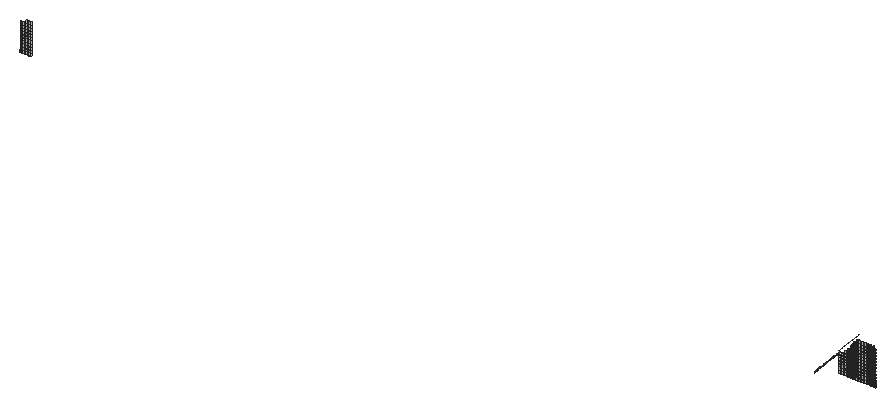
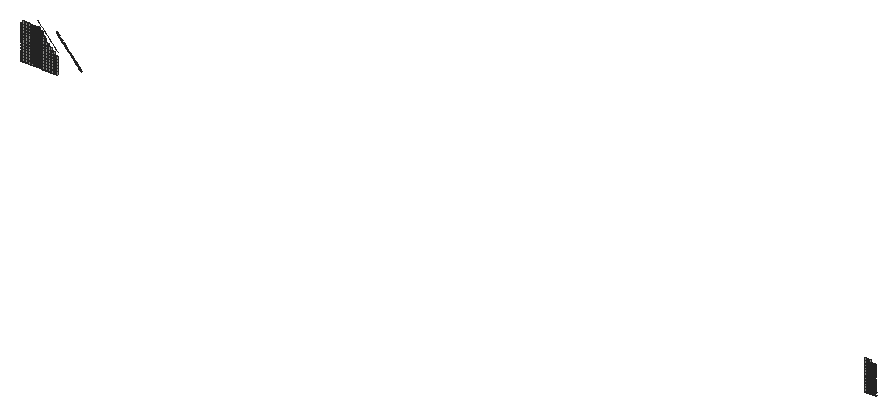
# SketchUp Ruby script. Lengths in inches.
U = 1.inch
M = Sketchup.active_model
def pt(a) = Geom::Point3d.new(a.map { |v| v * U })
def face(e, loops, mat)
  f = e.add_face(loops[0].map { |a| pt(a) })
  loops[1..].each { |l| e.add_face(l.map { |a| pt(a) }).erase! }
  f.material = f.back_material = mat if mat
  f
end
# faces: each face lists its corners as indices into pts; further lists are holes
def faces(e, pts, list, mat = nil) = list.each { |f| face(e, (f[0].is_a?(Array) ? f : [f]).map { |l| l.map { |i| pts[i] } }, mat) }
# xy, xz, yz: faces in a plane at the given z, y or x. An outline is a flat list of corners, or four numbers for a rectangle; further outlines are holes
def ring(l) = l.size == 4 ? [[l[0], l[1]], [l[2], l[1]], [l[2], l[3]], [l[0], l[3]]] : l.each_slice(2).to_a
def flat(e, list, mat, &to3) = list.each { |f| face(e, (f[0].is_a?(Array) ? f : [f]).map { |l| ring(l).map { |u, v| to3.(u, v) } }, mat) }
def xy(e, z, list, mat = nil) = flat(e, list, mat) { |x, y| [x, y, z] }
def xz(e, y, list, mat = nil) = flat(e, list, mat) { |x, z| [x, y, z] }
def yz(e, x, list, mat = nil) = flat(e, list, mat) { |y, z| [x, y, z] }
def lines(e, pts, list) = list.each { |a, b| e.add_line(pt(pts[a]), pt(pts[b])) }
# prism: a flat outline (further loops are holes) pulled along v
def prism(e, loops, v, mat = nil)
  f = face(e, loops, mat); d = Geom::Vector3d.new(v.map { |x| x * U })
  f.pushpull(f.normal.samedirection?(d) ? d.length : -d.length)
end
def box(e, o, s, mat = nil) = prism(e, [[o, [o[0] + s[0], o[1], o[2]], [o[0] + s[0], o[1] + s[1], o[2]], [o[0], o[1] + s[1], o[2]]]], [0, 0, s[2]], mat)
def at(x, y, z, deg = 0) = Geom::Transformation.translation(pt([x, y, z])) * Geom::Transformation.rotation(ORIGIN, Z_AXIS, deg.degrees)
def axes(o, x, y, z) = Geom::Transformation.new([*x, 0, *y, 0, *z, 0, *pt(o).to_a, 1])
def part(name) = M.definitions.add(name)
# library, detail: a bought-in or finely detailed component or shape, given as its bounding box
def library(name, o, s) = part(name).tap { |d| box(d.entities, o, s) }
def detail(e, o, s) = box(e.add_group.entities, o, s)
def put(e, d, t, mat = nil) = e.add_instance(d, t).tap { |i| i.material = mat if mat }
def group(e, t, mat = nil) = e.add_group.tap { |g| g.transformation = t; g.material = mat if mat }.entities
root = M.entities
M.materials.add("[Color M06]").color = [79, 71, 84]
xy(root,305.35,[[488.5,480.14,490.81,480.64],[491.41,480.14,493.72,480.77],[494.32,480.14,496.63,480.77],[497.23,480.14,499.55,480.77],[1319.63,480.14,1321.95,480.77],
  [1322.54,480.14,1324.86,480.77],[1325.46,480.14,1327.77,480.77],[1328.37,480.14,1330.68,480.77],[1331.28,480.14,1333.59,480.77],[1334.19,480.14,1336.51,480.77],
  [1337.11,480.14,1339.42,480.77],[1340.02,480.14,1342.33,480.77],[1342.93,480.14,1345.24,480.77],[1345.84,480.14,1348.15,480.77],[1348.75,480.14,1351.07,480.77],
  [1351.67,480.14,1353.98,480.77],[1354.58,480.14,1356.89,480.77]])
xy(root,307.67,[[488.5,480.14,490.81,480.64],[491.41,480.14,493.72,480.77],[494.32,480.14,496.63,480.77],[497.23,480.14,499.55,480.77],[1319.63,480.14,1321.95,480.77],
  [1322.54,480.14,1324.86,480.77],[1325.46,480.14,1327.77,480.77],[1328.37,480.14,1330.68,480.77],[1331.28,480.14,1333.59,480.77],[1334.19,480.14,1336.51,480.77],
  [1337.11,480.14,1339.42,480.77],[1340.02,480.14,1342.33,480.77],[1342.93,480.14,1345.24,480.77],[1345.84,480.14,1348.15,480.77],[1348.75,480.14,1351.07,480.77],
  [1351.67,480.14,1353.98,480.77],[1354.58,480.14,1356.89,480.77]])
xy(root,308.4,[[488.53,480.14,490.84,480.77],[491.4375,480.14,493.75,480.77],[494.35,480.14,496.66,480.77],[497.26,480.14,499.58,480.77],[1319.66,480.14,1321.97,480.77],
  [1322.57,480.14,1324.89,480.77],[1325.49,480.14,1327.8,480.77],[1328.4,480.14,1330.71,480.77],[1331.31,480.14,1333.62,480.77],[1334.22,480.14,1336.53,480.77],
  [1337.13,480.14,1339.45,480.77],[1340.05,480.14,1342.36,480.77],[1342.96,480.14,1345.27,480.77],[1345.87,480.14,1348.18,480.77],[1348.78,480.14,1351.09,480.77],
  [1351.69,480.14,1354.01,480.77],[1354.61,480.14,1356.92,480.77]])
xy(root,310.71,[[488.53,480.14,490.84,480.77],[491.4375,480.14,493.75,480.77],[494.35,480.14,496.66,480.77],[497.26,480.14,499.58,480.77],[1319.66,480.14,1321.97,480.77],
  [1322.57,480.14,1324.89,480.77],[1325.49,480.14,1327.8,480.77],[1328.4,480.14,1330.71,480.77],[1331.31,480.14,1333.62,480.77],[1334.22,480.14,1336.53,480.77],
  [1337.13,480.14,1339.45,480.77],[1340.05,480.14,1342.36,480.77],[1342.96,480.14,1345.27,480.77],[1345.87,480.14,1348.18,480.77],[1348.78,480.14,1351.09,480.77],
  [1351.69,480.14,1354.01,480.77],[1354.61,480.14,1356.92,480.77]])
xy(root,311.21,[[488.53,480.14,490.84,480.77],[491.4375,480.14,493.75,480.77],[494.35,480.14,496.66,480.77],[497.26,480.14,499.58,480.77],[1319.66,480.14,1321.97,480.77],
  [1322.57,480.14,1324.89,480.77],[1325.49,480.14,1327.8,480.77],[1328.4,480.14,1330.71,480.77],[1331.31,480.14,1333.62,480.77],[1334.22,480.14,1336.53,480.77],
  [1337.13,480.14,1339.45,480.77],[1340.05,480.14,1342.36,480.77],[1342.96,480.14,1345.27,480.77],[1345.87,480.14,1348.18,480.77],[1348.78,480.14,1351.09,480.77],
  [1351.69,480.14,1354.01,480.77],[1354.61,480.14,1356.92,480.77]])
xy(root,313.52,[[488.53,480.14,490.84,480.77],[491.4375,480.14,493.75,480.77],[494.35,480.14,496.66,480.77],[497.26,480.14,499.58,480.77],[1319.66,480.14,1321.97,480.77],
  [1322.57,480.14,1324.89,480.77],[1325.49,480.14,1327.8,480.77],[1328.4,480.14,1330.71,480.77],[1331.31,480.14,1333.62,480.77],[1334.22,480.14,1336.53,480.77],
  [1337.13,480.14,1339.45,480.77],[1340.05,480.14,1342.36,480.77],[1342.96,480.14,1345.27,480.77],[1345.87,480.14,1348.18,480.77],[1348.78,480.14,1351.09,480.77],
  [1351.69,480.14,1354.01,480.77],[1354.61,480.14,1356.92,480.77]])
xy(root,314.02,[[488.53,480.14,490.84,480.77],[491.4375,480.14,493.75,480.77],[494.35,480.14,496.66,480.77],[497.26,480.14,499.58,480.77],[1319.66,480.14,1321.97,480.77],
  [1322.57,480.14,1324.89,480.77],[1325.49,480.14,1327.8,480.77],[1328.4,480.14,1330.71,480.77],[1331.31,480.14,1333.62,480.77],[1334.22,480.14,1336.53,480.77],
  [1337.13,480.14,1339.45,480.77],[1340.05,480.14,1342.36,480.77],[1342.96,480.14,1345.27,480.77],[1345.87,480.14,1348.18,480.77],[1348.78,480.14,1351.09,480.77],
  [1351.69,480.14,1354.01,480.77],[1354.61,480.14,1356.92,480.77]])
xy(root,316.34,[[488.53,480.14,490.84,480.77],[491.4375,480.14,493.75,480.77],[494.35,480.14,496.66,480.77],[497.26,480.14,499.58,480.77],[1319.66,480.14,1321.97,480.77],
  [1322.57,480.14,1324.89,480.77],[1325.49,480.14,1327.8,480.77],[1328.4,480.14,1330.71,480.77],[1331.31,480.14,1333.62,480.77],[1334.22,480.14,1336.53,480.77],
  [1337.13,480.14,1339.45,480.77],[1340.05,480.14,1342.36,480.77],[1342.96,480.14,1345.27,480.77],[1345.87,480.14,1348.18,480.77],[1348.78,480.14,1351.09,480.77],
  [1351.69,480.14,1354.01,480.77],[1354.61,480.14,1356.92,480.77]])
xy(root,316.84,[[488.53,480.14,490.84,480.77],[491.4375,480.14,493.75,480.77],[494.35,480.14,496.66,480.77],[497.26,480.14,499.58,480.77],[1319.66,480.14,1321.97,480.77],
  [1322.57,480.14,1324.89,480.77],[1325.49,480.14,1327.8,480.77],[1328.4,480.14,1330.71,480.77],[1331.31,480.14,1333.62,480.77],[1334.22,480.14,1336.53,480.77],
  [1337.13,480.14,1339.45,480.77],[1340.05,480.14,1342.36,480.77],[1342.96,480.14,1345.27,480.77],[1345.87,480.14,1348.18,480.77],[1348.78,480.14,1351.09,480.77],
  [1351.69,480.14,1354.01,480.77],[1354.61,480.14,1356.92,480.77]])
xy(root,319.15,[[488.53,480.14,490.84,480.77],[491.4375,480.14,493.75,480.77],[494.35,480.14,496.66,480.77],[497.26,480.14,499.58,480.77],[1319.66,480.14,1321.97,480.77],
  [1322.57,480.14,1324.89,480.77],[1325.49,480.14,1327.8,480.77],[1328.4,480.14,1330.71,480.77],[1331.31,480.14,1333.62,480.77],[1334.22,480.14,1336.53,480.77],
  [1337.13,480.14,1339.45,480.77],[1340.05,480.14,1342.36,480.77],[1342.96,480.14,1345.27,480.77],[1345.87,480.14,1348.18,480.77],[1348.78,480.14,1351.09,480.77],
  [1351.69,480.14,1354.01,480.77],[1354.61,480.14,1356.92,480.77]])
xy(root,319.65,[[488.53,480.14,490.84,480.7],[491.4375,480.14,493.75,480.7],[494.35,480.14,496.66,480.7],[497.26,480.14,499.58,480.77],[1319.66,480.14,1321.97,480.77],
  [1322.57,480.14,1324.89,480.77],[1325.49,480.14,1327.8,480.77],[1328.4,480.14,1330.71,480.77],[1331.31,480.14,1333.62,480.77],[1334.22,480.14,1336.53,480.77],
  [1337.13,480.14,1339.45,480.77],[1340.05,480.14,1342.36,480.77],[1342.96,480.14,1345.27,480.77],[1345.87,480.14,1348.18,480.77],[1348.78,480.14,1351.09,480.77],
  [1351.69,480.14,1354.01,480.77],[1354.61,480.14,1356.92,480.77]])
xy(root,321.96,[[488.53,480.14,490.84,480.7],[491.4375,480.14,493.75,480.7],[494.35,480.14,496.66,480.7],[497.26,480.14,499.58,480.77],[1320.19,480.14,1321.97,480.77],
  [1322.57,480.14,1324.89,480.77],[1325.49,480.14,1327.8,480.77],[1328.4,480.14,1330.71,480.77],[1331.31,480.14,1333.62,480.77],[1334.22,480.14,1336.53,480.77],
  [1337.13,480.14,1339.45,480.77],[1340.05,480.14,1342.36,480.77],[1342.96,480.14,1345.27,480.77],[1345.87,480.14,1348.18,480.77],[1348.78,480.14,1351.09,480.77],
  [1351.69,480.14,1354.01,480.77],[1354.61,480.14,1356.92,480.77]])
xy(root,322.46,[[488.53,480.14,490.84,480.77],[491.4375,480.14,493.75,480.77],[494.35,480.14,496.66,480.77],[497.26,480.14,499.58,480.77],[1322.57,480.14,1324.89,480.77],
  [1325.49,480.14,1327.8,480.77],[1328.4,480.14,1330.71,480.77],[1331.31,480.14,1333.62,480.77],[1334.22,480.14,1336.53,480.77],[1337.13,480.14,1339.45,480.77],
  [1340.05,480.14,1342.36,480.77],[1342.96,480.14,1345.27,480.77],[1345.87,480.14,1348.18,480.77],[1348.78,480.14,1351.09,480.77],[1351.69,480.14,1354.01,480.77],
  [1354.61,480.14,1356.92,480.77]])
xy(root,324.77,[[488.53,480.14,490.84,480.77],[491.4375,480.14,493.75,480.77],[494.35,480.14,496.66,480.77],[497.26,480.14,499.58,480.77],[1322.83,480.14,1324.89,480.77],
  [1325.49,480.14,1327.8,480.77],[1328.4,480.14,1330.71,480.77],[1331.31,480.14,1333.62,480.77],[1334.22,480.14,1336.53,480.77],[1337.13,480.14,1339.45,480.77],
  [1340.05,480.14,1342.36,480.77],[1342.96,480.14,1345.27,480.77],[1345.87,480.14,1348.18,480.77],[1348.78,480.14,1351.09,480.77],[1351.69,480.14,1354.01,480.77],
  [1354.61,480.14,1356.92,480.77]])
xy(root,325.27,[[488.53,480.14,490.84,480.77],[491.4375,480.14,493.75,480.77],[494.35,480.14,496.66,480.77],[497.26,480.14,499.58,480.77],[1325.49,480.14,1327.8,480.77],
  [1328.4,480.14,1330.71,480.77],[1331.31,480.14,1333.62,480.77],[1334.22,480.14,1336.53,480.77],[1337.13,480.14,1339.45,480.77],[1340.05,480.14,1342.36,480.77],
  [1342.96,480.14,1345.27,480.77],[1345.87,480.14,1348.18,480.77],[1348.78,480.14,1351.09,480.77],[1351.69,480.14,1354.01,480.77],[1354.61,480.14,1356.92,480.77]])
xy(root,327.59,[[488.53,480.14,490.84,480.77],[491.4375,480.14,493.75,480.77],[494.35,480.14,496.66,480.77],[497.26,480.14,499.58,480.77],[1325.49,480.14,1327.8,480.77],
  [1328.4,480.14,1330.71,480.77],[1331.31,480.14,1333.62,480.77],[1334.22,480.14,1336.53,480.77],[1337.13,480.14,1339.45,480.77],[1340.05,480.14,1342.36,480.77],
  [1342.96,480.14,1345.27,480.77],[1345.87,480.14,1348.18,480.77],[1348.78,480.14,1351.09,480.77],[1351.69,480.14,1354.01,480.77],[1354.61,480.14,1356.92,480.77]])
xy(root,328.09,[[488.53,480.14,490.84,480.77],[491.4375,480.14,493.75,480.77],[494.35,480.14,496.66,480.77],[497.26,480.14,499.58,480.77],[1328.4,480.14,1330.71,480.77],
  [1331.31,480.14,1333.62,480.77],[1334.22,480.14,1336.53,480.77],[1337.13,480.14,1339.45,480.77],[1340.05,480.14,1342.36,480.77],[1342.96,480.14,1345.27,480.77],
  [1345.87,480.14,1348.18,480.77],[1348.78,480.14,1351.09,480.77],[1351.69,480.14,1354.01,480.77],[1354.61,480.14,1356.92,480.77]])
xy(root,330.4,[[488.53,480.14,490.84,480.77],[491.4375,480.14,493.75,480.77],[494.35,480.14,496.66,480.77],[497.26,480.14,499.58,480.77],[1328.4,480.14,1330.71,480.77],
  [1331.31,480.14,1333.62,480.77],[1334.22,480.14,1336.53,480.77],[1337.13,480.14,1339.45,480.77],[1340.05,480.14,1342.36,480.77],[1342.96,480.14,1345.27,480.77],
  [1345.87,480.14,1348.18,480.77],[1348.78,480.14,1351.09,480.77],[1351.69,480.14,1354.01,480.77],[1354.61,480.14,1356.92,480.77]])
xy(root,330.9,[[488.53,480.14,490.84,480.77],[491.4375,480.14,493.75,480.77],[494.35,480.14,496.66,480.77],[497.26,480.14,499.58,480.77],[1331.31,480.14,1333.62,480.77],
  [1334.22,480.14,1336.53,480.77],[1337.13,480.14,1339.45,480.77],[1340.05,480.14,1342.36,480.77],[1342.96,480.14,1345.27,480.77],[1345.87,480.14,1348.18,480.77],
  [1348.78,480.14,1351.09,480.77],[1351.69,480.14,1354.01,480.77],[1354.61,480.14,1356.92,480.77]])
xy(root,333.21,[[488.53,480.14,490.84,480.77],[491.4375,480.14,493.75,480.77],[494.35,480.14,496.66,480.77],[497.26,480.14,499.58,480.77],[1331.31,480.14,1333.62,480.77],
  [1334.22,480.14,1336.53,480.77],[1337.13,480.14,1339.45,480.77],[1340.05,480.14,1342.36,480.77],[1342.96,480.14,1345.27,480.77],[1345.87,480.14,1348.18,480.77],
  [1348.78,480.14,1351.09,480.77],[1351.69,480.14,1354.01,480.77],[1354.61,480.14,1356.92,480.77]])
xy(root,333.71,[[1331.31,480.14,1333.62,480.77],[1334.22,480.14,1336.53,480.77],[1337.13,480.14,1339.45,480.77],[1340.05,480.14,1342.36,480.77],[1342.96,480.14,1345.27,480.77],
  [1345.87,480.14,1348.18,480.77],[1348.78,480.14,1351.09,480.77],[1351.69,480.14,1354.01,480.77],[1354.61,480.14,1356.92,480.77]])
xy(root,336.02,[[1333.375,480.14,1333.62,480.77],[1334.22,480.14,1336.53,480.77],[1337.13,480.14,1339.45,480.77],[1340.05,480.14,1342.36,480.77],[1342.96,480.14,1345.27,480.77],
  [1345.87,480.14,1348.18,480.77],[1348.78,480.14,1351.09,480.77],[1351.69,480.14,1354.01,480.77],[1354.61,480.14,1356.92,480.77]])
xy(root,336.52,[[1334.22,480.14,1336.53,480.77],[1337.13,480.14,1339.45,480.77],[1340.05,480.14,1342.36,480.77],[1342.96,480.14,1345.27,480.77],[1345.87,480.14,1348.18,480.77],
  [1348.78,480.14,1351.09,480.77],[1351.69,480.14,1354.01,480.77],[1354.61,480.14,1356.92,480.77]])
xy(root,338.84,[[1336.01,480.14,1336.53,480.77],[1337.13,480.14,1339.45,480.77],[1340.05,480.14,1342.36,480.77],[1342.96,480.14,1345.27,480.77],[1345.87,480.14,1348.18,480.77],
  [1348.78,480.14,1351.09,480.77],[1351.69,480.14,1354.01,480.77],[1354.61,480.14,1356.92,480.77]])
xy(root,339.34,[[1337.13,480.14,1339.45,480.77],[1340.05,480.14,1342.36,480.77],[1342.96,480.14,1345.27,480.77],[1345.87,480.14,1348.18,480.77],[1348.78,480.14,1351.09,480.77],
  [1351.69,480.14,1354.01,480.77],[1354.61,480.14,1356.92,480.77]])
xz(root,467.1875,[[1305.53,306.65,1307.95,309.22,1307.5,309.65,1305.08,307.08],[1305.08,307.08,1307.5,309.65,1307.27,309.87,1304.85,307.29],[1308.83,310.16,1311.25,312.73,1310.8,313.16,1308.375,310.59],[1312.13,313.66,1314.55,316.23,1314.1,316.66,1311.68,314.09],[1315.43,317.17,1317.85,319.74,1317.39,320.17,1314.97,317.59],
  [1318.73,320.67,1321.15,323.24,1320.69,323.67,1318.27,321.1],[1322.03,324.17,1324.45,326.75,1323.99,327.17,1321.57,324.6],[1325.32,327.68,1327.75,330.25,1327.29,330.68,1324.87,328.11],[1328.62,331.18,1331.04,333.75,1330.59,334.18,1328.17,331.61]],"[Color M06]")
xz(root,480.14,[[1322.57,324.5,1322.83,324.77,1322.57,324.77],[1334.22,336.93,1336.01,338.84,1334.22,338.84],[1337.13,340.04,1338.65,341.65,1337.13,341.65]])
yz(root,488.53,[[480.14,308.4,480.77,310.71],[480.14,311.21,480.77,313.52],[480.14,314.02,480.77,316.34],[480.14,316.84,480.77,319.15],[480.14,322.46,480.77,324.77],
  [480.14,325.27,480.77,327.59],[480.14,328.09,480.77,330.4],[480.14,330.9,480.77,333.21]])
yz(root,490.81,[[480.14,305.35,480.64,307.67]])
yz(root,490.84,[[480.14,308.4,480.77,310.71],[480.14,311.21,480.77,313.52],[480.14,314.02,480.77,316.34],[480.14,316.84,480.77,319.15],[480.14,319.65,480.7,321.96],
  [480.14,322.46,480.77,324.77],[480.14,325.27,480.77,327.59],[480.14,328.09,480.77,330.4],[480.14,330.9,480.77,333.21]])
yz(root,491.41,[[480.14,305.35,480.77,307.67]])
yz(root,491.4375,[[480.14,308.4,480.77,310.71],[480.14,311.21,480.77,313.52],[480.14,314.02,480.77,316.34],[480.14,316.84,480.77,319.15],[480.14,319.65,480.7,321.96],
  [480.14,322.46,480.77,324.77],[480.14,325.27,480.77,327.59],[480.14,328.09,480.77,330.4],[480.14,330.9,480.77,333.21]])
yz(root,493.72,[[480.14,305.35,480.77,307.67]])
yz(root,493.75,[[480.14,308.4,480.77,310.71],[480.14,311.21,480.77,313.52],[480.14,314.02,480.77,316.34],[480.14,316.84,480.77,319.15],[480.14,319.65,480.7,321.96],
  [480.14,322.46,480.77,324.77],[480.14,325.27,480.77,327.59],[480.14,328.09,480.77,330.4],[480.14,330.9,480.77,333.21]])
yz(root,494.32,[[480.14,305.35,480.77,307.67]])
yz(root,494.35,[[480.14,308.4,480.77,310.71],[480.14,311.21,480.77,313.52],[480.14,314.02,480.77,316.34],[480.14,316.84,480.77,319.15],[480.14,319.65,480.7,321.96],
  [480.14,322.46,480.77,324.77],[480.14,325.27,480.77,327.59],[480.14,328.09,480.77,330.4],[480.14,330.9,480.77,333.21],[480.14,333.71,480.77,336.02]])
yz(root,496.63,[[480.14,305.35,480.77,307.67]])
yz(root,496.66,[[480.14,308.4,480.77,310.71],[480.14,311.21,480.77,313.52],[480.14,314.02,480.77,316.34],[480.14,316.84,480.77,319.15],[480.14,319.65,480.7,321.96],
  [480.14,322.46,480.77,324.77],[480.14,325.27,480.77,327.59],[480.14,328.09,480.77,330.4],[480.14,330.9,480.77,333.21],[480.14,333.71,480.77,336.02]])
yz(root,497.23,[[480.14,305.35,480.77,307.67]])
yz(root,497.26,[[480.14,308.4,480.77,310.71],[480.14,311.21,480.77,313.52],[480.14,314.02,480.77,316.34],[480.14,316.84,480.77,319.15],[480.14,319.65,480.77,321.96],
  [480.14,322.46,480.77,324.77],[480.14,325.27,480.77,327.59],[480.14,328.09,480.77,330.4],[480.14,330.9,480.77,333.21],[480.14,333.71,480.77,336.02]])
yz(root,499.55,[[480.14,305.35,480.77,307.67]])
yz(root,499.58,[[480.14,308.4,480.77,310.71],[480.14,311.21,480.77,313.52],[480.14,314.02,480.77,316.34],[480.14,316.84,480.77,319.15],[480.14,319.65,480.77,321.96],
  [480.14,322.46,480.77,324.77],[480.14,325.27,480.77,327.59],[480.14,328.09,480.77,330.4],[480.14,330.9,480.77,333.21],[480.14,333.71,480.77,336.02]])
yz(root,1319.63,[[480.14,305.35,480.77,307.67]])
yz(root,1319.66,[[480.14,308.4,480.77,310.71],[480.14,311.21,480.77,313.52],[480.14,314.02,480.77,316.34],[480.14,316.84,480.77,319.15],[480.14,319.65,480.77,321.39]])
yz(root,1321.95,[[480.14,305.35,480.77,307.67]])
yz(root,1321.97,[[480.14,308.4,480.77,310.71],[480.14,311.21,480.77,313.52],[480.14,314.02,480.77,316.34],[480.14,316.84,480.77,319.15],[480.14,319.65,480.77,321.96]])
yz(root,1322.54,[[480.14,305.35,480.77,307.67]])
yz(root,1322.57,[[480.14,308.4,480.77,310.71],[480.14,311.21,480.77,313.52],[480.14,314.02,480.77,316.34],[480.14,316.84,480.77,319.15],[480.14,319.65,480.77,321.96],
  [480.14,322.46,480.77,324.5]])
yz(root,1324.86,[[480.14,305.35,480.77,307.67]])
yz(root,1324.89,[[480.14,308.4,480.77,310.71],[480.14,311.21,480.77,313.52],[480.14,314.02,480.77,316.34],[480.14,316.84,480.77,319.15],[480.14,319.65,480.77,321.96],
  [480.14,322.46,480.77,324.77]])
yz(root,1325.46,[[480.14,305.35,480.77,307.67]])
yz(root,1325.49,[[480.14,308.4,480.77,310.71],[480.14,311.21,480.77,313.52],[480.14,314.02,480.77,316.34],[480.14,316.84,480.77,319.15],[480.14,319.65,480.77,321.96],
  [480.14,322.46,480.77,324.77],[480.14,325.27,480.77,327.59]])
yz(root,1327.77,[[480.14,305.35,480.77,307.67]])
yz(root,1327.8,[[480.14,308.4,480.77,310.71],[480.14,311.21,480.77,313.52],[480.14,314.02,480.77,316.34],[480.14,316.84,480.77,319.15],[480.14,319.65,480.77,321.96],
  [480.14,322.46,480.77,324.77],[480.14,325.27,480.77,327.59]])
yz(root,1328.37,[[480.14,305.35,480.77,307.67]])
yz(root,1328.4,[[480.14,308.4,480.77,310.71],[480.14,311.21,480.77,313.52],[480.14,314.02,480.77,316.34],[480.14,316.84,480.77,319.15],[480.14,319.65,480.77,321.96],
  [480.14,322.46,480.77,324.77],[480.14,325.27,480.77,327.59],[480.14,328.09,480.77,330.4]])
yz(root,1330.68,[[480.14,305.35,480.77,307.67]])
yz(root,1330.71,[[480.14,308.4,480.77,310.71],[480.14,311.21,480.77,313.52],[480.14,314.02,480.77,316.34],[480.14,316.84,480.77,319.15],[480.14,319.65,480.77,321.96],
  [480.14,322.46,480.77,324.77],[480.14,325.27,480.77,327.59],[480.14,328.09,480.77,330.4]])
yz(root,1331.28,[[480.14,305.35,480.77,307.67]])
yz(root,1331.31,[[480.14,308.4,480.77,310.71],[480.14,311.21,480.77,313.52],[480.14,314.02,480.77,316.34],[480.14,316.84,480.77,319.15],[480.14,319.65,480.77,321.96],
  [480.14,322.46,480.77,324.77],[480.14,325.27,480.77,327.59],[480.14,328.09,480.77,330.4],[480.14,330.9,480.77,333.21],[480.14,333.71,480.77,333.82]])
yz(root,1333.59,[[480.14,305.35,480.77,307.67]])
yz(root,1333.62,[[480.14,308.4,480.77,310.71],[480.14,311.21,480.77,313.52],[480.14,314.02,480.77,316.34],[480.14,316.84,480.77,319.15],[480.14,319.65,480.77,321.96],
  [480.14,322.46,480.77,324.77],[480.14,325.27,480.77,327.59],[480.14,328.09,480.77,330.4],[480.14,330.9,480.77,333.21],[480.14,333.71,480.77,336.02]])
yz(root,1334.19,[[480.14,305.35,480.77,307.67]])
yz(root,1334.22,[[480.14,308.4,480.77,310.71],[480.14,311.21,480.77,313.52],[480.14,314.02,480.77,316.34],[480.14,316.84,480.77,319.15],[480.14,319.65,480.77,321.96],
  [480.14,322.46,480.77,324.77],[480.14,325.27,480.77,327.59],[480.14,328.09,480.77,330.4],[480.14,330.9,480.77,333.21],[480.14,333.71,480.77,336.02],
  [480.14,336.52,480.77,336.93]])
yz(root,1336.51,[[480.14,305.35,480.77,307.67]])
yz(root,1336.53,[[480.14,308.4,480.77,310.71],[480.14,311.21,480.77,313.52],[480.14,314.02,480.77,316.34],[480.14,316.84,480.77,319.15],[480.14,319.65,480.77,321.96],
  [480.14,322.46,480.77,324.77],[480.14,325.27,480.77,327.59],[480.14,328.09,480.77,330.4],[480.14,330.9,480.77,333.21],[480.14,333.71,480.77,336.02],
  [480.14,336.52,480.77,338.84]])
yz(root,1337.11,[[480.14,305.35,480.77,307.67]])
yz(root,1337.13,[[480.14,308.4,480.77,310.71],[480.14,311.21,480.77,313.52],[480.14,314.02,480.77,316.34],[480.14,316.84,480.77,319.15],[480.14,319.65,480.77,321.96],
  [480.14,322.46,480.77,324.77],[480.14,325.27,480.77,327.59],[480.14,328.09,480.77,330.4],[480.14,330.9,480.77,333.21],[480.14,333.71,480.77,336.02],
  [480.14,336.52,480.77,338.84],[480.14,339.34,480.77,340.04]])
yz(root,1339.42,[[480.14,305.35,480.77,307.67]])
yz(root,1339.45,[[480.14,308.4,480.77,310.71],[480.14,311.21,480.77,313.52],[480.14,314.02,480.77,316.34],[480.14,316.84,480.77,319.15],[480.14,319.65,480.77,321.96],
  [480.14,322.46,480.77,324.77],[480.14,325.27,480.77,327.59],[480.14,328.09,480.77,330.4],[480.14,330.9,480.77,333.21],[480.14,333.71,480.77,336.02],
  [480.14,336.52,480.77,338.84],[480.14,339.34,480.77,341.65]])
yz(root,1340.02,[[480.14,305.35,480.77,307.67]])
yz(root,1340.05,[[480.14,308.4,480.77,310.71],[480.14,311.21,480.77,313.52],[480.14,314.02,480.77,316.34],[480.14,316.84,480.77,319.15],[480.14,319.65,480.77,321.96],
  [480.14,322.46,480.77,324.77],[480.14,325.27,480.77,327.59],[480.14,328.09,480.77,330.4],[480.14,330.9,480.77,333.21],[480.14,333.71,480.77,336.02],
  [480.14,336.52,480.77,338.84],[480.14,339.34,480.77,341.65]])
yz(root,1342.33,[[480.14,305.35,480.77,307.67]])
yz(root,1342.36,[[480.14,308.4,480.77,310.71],[480.14,311.21,480.77,313.52],[480.14,314.02,480.77,316.34],[480.14,316.84,480.77,319.15],[480.14,319.65,480.77,321.96],
  [480.14,322.46,480.77,324.77],[480.14,325.27,480.77,327.59],[480.14,328.09,480.77,330.4],[480.14,330.9,480.77,333.21],[480.14,333.71,480.77,336.02],
  [480.14,336.52,480.77,338.84],[480.14,339.34,480.77,341.65]])
yz(root,1342.93,[[480.14,305.35,480.77,307.67]])
yz(root,1342.96,[[480.14,308.4,480.77,310.71],[480.14,311.21,480.77,313.52],[480.14,314.02,480.77,316.34],[480.14,316.84,480.77,319.15],[480.14,319.65,480.77,321.96],
  [480.14,322.46,480.77,324.77],[480.14,325.27,480.77,327.59],[480.14,328.09,480.77,330.4],[480.14,330.9,480.77,333.21],[480.14,333.71,480.77,336.02],
  [480.14,336.52,480.77,338.84],[480.14,339.34,480.77,341.65]])
yz(root,1345.24,[[480.14,305.35,480.77,307.67]])
yz(root,1345.27,[[480.14,308.4,480.77,310.71],[480.14,311.21,480.77,313.52],[480.14,314.02,480.77,316.34],[480.14,316.84,480.77,319.15],[480.14,319.65,480.77,321.96],
  [480.14,322.46,480.77,324.77],[480.14,325.27,480.77,327.59],[480.14,328.09,480.77,330.4],[480.14,330.9,480.77,333.21],[480.14,333.71,480.77,336.02],
  [480.14,336.52,480.77,338.84],[480.14,339.34,480.77,341.65]])
yz(root,1345.84,[[480.14,305.35,480.77,307.67]])
yz(root,1345.87,[[480.14,308.4,480.77,310.71],[480.14,311.21,480.77,313.52],[480.14,314.02,480.77,316.34],[480.14,316.84,480.77,319.15],[480.14,319.65,480.77,321.96],
  [480.14,322.46,480.77,324.77],[480.14,325.27,480.77,327.59],[480.14,328.09,480.77,330.4],[480.14,330.9,480.77,333.21],[480.14,333.71,480.77,336.02],
  [480.14,336.52,480.77,338.84],[480.14,339.34,480.77,341.65]])
yz(root,1348.15,[[480.14,305.35,480.77,307.67]])
yz(root,1348.18,[[480.14,308.4,480.77,310.71],[480.14,311.21,480.77,313.52],[480.14,314.02,480.77,316.34],[480.14,316.84,480.77,319.15],[480.14,319.65,480.77,321.96],
  [480.14,322.46,480.77,324.77],[480.14,325.27,480.77,327.59],[480.14,328.09,480.77,330.4],[480.14,330.9,480.77,333.21],[480.14,333.71,480.77,336.02],
  [480.14,336.52,480.77,338.84],[480.14,339.34,480.77,341.65]])
yz(root,1348.75,[[480.14,305.35,480.77,307.67]])
yz(root,1348.78,[[480.14,308.4,480.77,310.71],[480.14,311.21,480.77,313.52],[480.14,314.02,480.77,316.34],[480.14,316.84,480.77,319.15],[480.14,319.65,480.77,321.96],
  [480.14,322.46,480.77,324.77],[480.14,325.27,480.77,327.59],[480.14,328.09,480.77,330.4],[480.14,330.9,480.77,333.21],[480.14,333.71,480.77,336.02],
  [480.14,336.52,480.77,338.84],[480.14,339.34,480.77,341.65]])
yz(root,1351.07,[[480.14,305.35,480.77,307.67]])
yz(root,1351.09,[[480.14,308.4,480.77,310.71],[480.14,311.21,480.77,313.52],[480.14,314.02,480.77,316.34],[480.14,316.84,480.77,319.15],[480.14,319.65,480.77,321.96],
  [480.14,322.46,480.77,324.77],[480.14,325.27,480.77,327.59],[480.14,328.09,480.77,330.4],[480.14,330.9,480.77,333.21],[480.14,333.71,480.77,336.02],
  [480.14,336.52,480.77,338.84],[480.14,339.34,480.77,341.65]])
yz(root,1351.67,[[480.14,305.35,480.77,307.67]])
yz(root,1351.69,[[480.14,308.4,480.77,310.71],[480.14,311.21,480.77,313.52],[480.14,314.02,480.77,316.34],[480.14,316.84,480.77,319.15],[480.14,319.65,480.77,321.96],
  [480.14,322.46,480.77,324.77],[480.14,325.27,480.77,327.59],[480.14,328.09,480.77,330.4],[480.14,330.9,480.77,333.21],[480.14,333.71,480.77,336.02],
  [480.14,336.52,480.77,338.84],[480.14,339.34,480.77,341.65]])
yz(root,1353.98,[[480.14,305.35,480.77,307.67]])
yz(root,1354.01,[[480.14,308.4,480.77,310.71],[480.14,311.21,480.77,313.52],[480.14,314.02,480.77,316.34],[480.14,316.84,480.77,319.15],[480.14,319.65,480.77,321.96],
  [480.14,322.46,480.77,324.77],[480.14,325.27,480.77,327.59],[480.14,328.09,480.77,330.4],[480.14,330.9,480.77,333.21],[480.14,333.71,480.77,336.02],
  [480.14,336.52,480.77,338.84],[480.14,339.34,480.77,341.65]])
yz(root,1354.58,[[480.14,305.35,480.77,307.67]])
yz(root,1354.61,[[480.14,308.4,480.77,310.71],[480.14,311.21,480.77,313.52],[480.14,314.02,480.77,316.34],[480.14,316.84,480.77,319.15],[480.14,319.65,480.77,321.96],
  [480.14,322.46,480.77,324.77],[480.14,325.27,480.77,327.59],[480.14,328.09,480.77,330.4],[480.14,330.9,480.77,333.21],[480.14,333.71,480.77,336.02],
  [480.14,336.52,480.77,338.84],[480.14,339.34,480.77,341.65]])
yz(root,1356.89,[[480.14,305.35,480.77,307.67]])
yz(root,1356.92,[[480.14,308.4,480.77,310.71]])
p = [[1320.19,480.14,321.96],[1319.66,480.14,321.39],[1319.66,480.77,321.39],[1320.19,480.77,321.96],[1322.83,480.14,324.77],[1322.57,480.14,324.5],
  [1322.57,480.77,324.5],[1322.83,480.77,324.77],[1333.375,480.14,336.02],[1331.31,480.14,333.82],[1331.31,480.77,333.82],[1333.375,480.77,336.02],
  [1336.01,480.14,338.84],[1334.22,480.14,336.93],[1334.22,480.77,336.93],[1336.01,480.77,338.84],[1338.65,480.14,341.65],[1337.13,480.14,340.04],
  [1337.13,480.77,340.04],[1338.65,480.77,341.65],[1340.05,480.14,347.77],[1319.33,480.14,325.75]]
faces(root,p,[[0,1,2,3],[4,5,6,7],[8,9,10,11],[12,13,14,15],[16,17,18,19]])
lines(root,p,[[20,21]])
